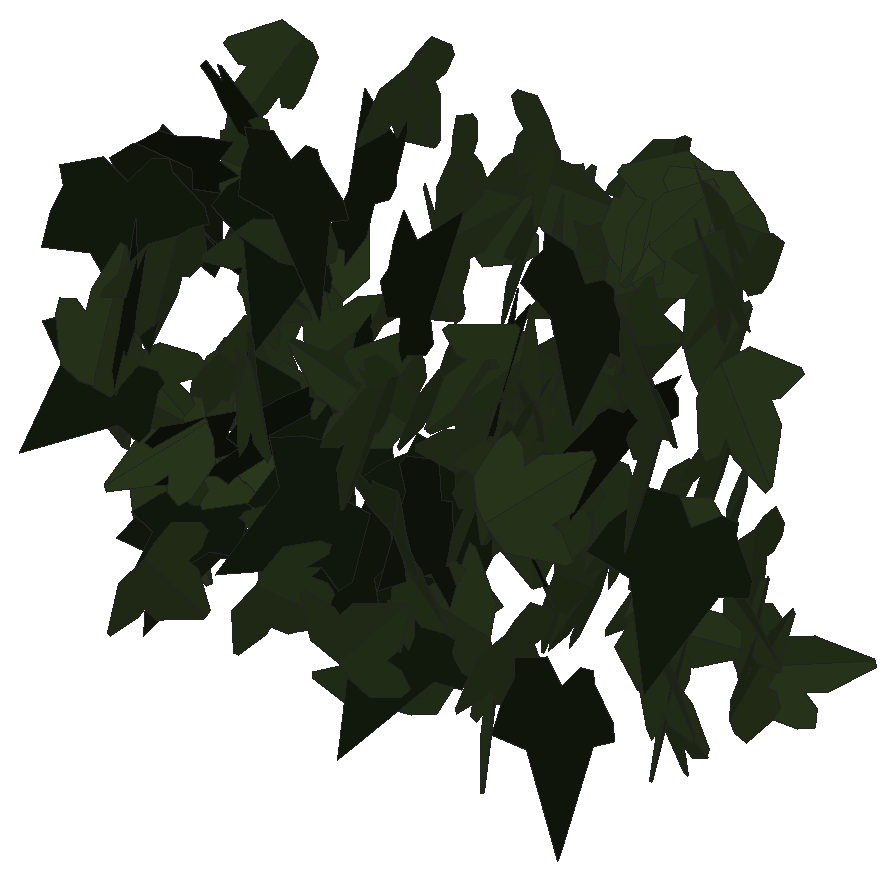
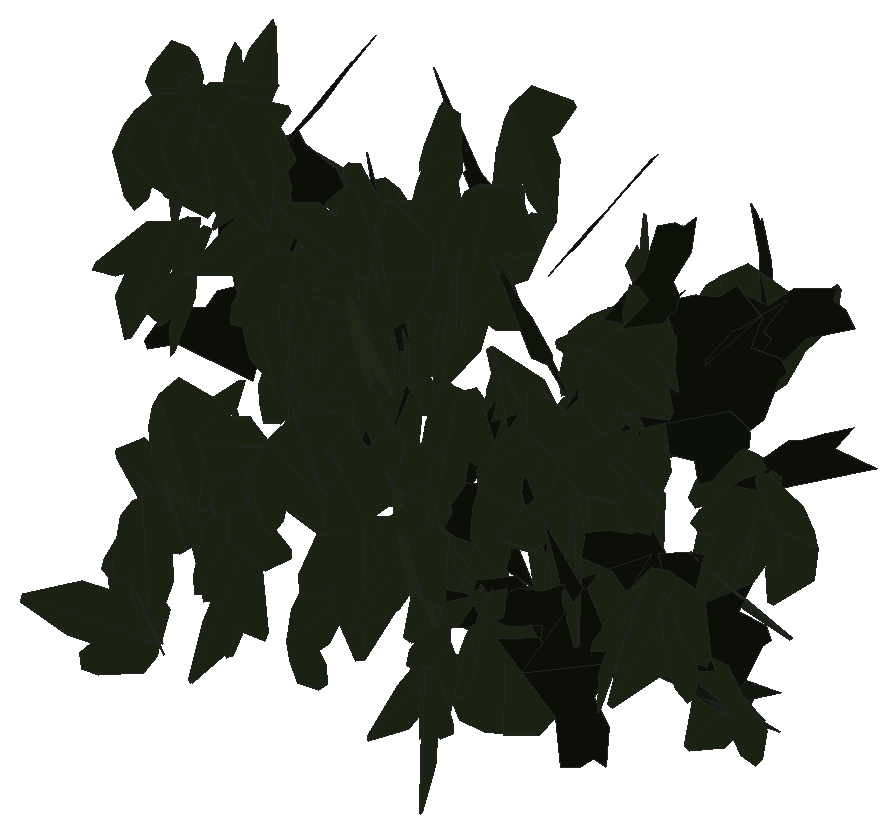
# SketchUp Ruby script. Lengths in inches.
U = 1.inch
M = Sketchup.active_model
def pt(a) = Geom::Point3d.new(a.map { |v| v * U })
def face(e, loops, mat)
  f = e.add_face(loops[0].map { |a| pt(a) })
  loops[1..].each { |l| e.add_face(l.map { |a| pt(a) }).erase! }
  f.material = f.back_material = mat if mat
  f
end
# faces: each face lists its corners as indices into pts; further lists are holes
def faces(e, pts, list, mat = nil) = list.each { |f| face(e, (f[0].is_a?(Array) ? f : [f]).map { |l| l.map { |i| pts[i] } }, mat) }
# xy, xz, yz: faces in a plane at the given z, y or x. An outline is a flat list of corners, or four numbers for a rectangle; further outlines are holes
def ring(l) = l.size == 4 ? [[l[0], l[1]], [l[2], l[1]], [l[2], l[3]], [l[0], l[3]]] : l.each_slice(2).to_a
def flat(e, list, mat, &to3) = list.each { |f| face(e, (f[0].is_a?(Array) ? f : [f]).map { |l| ring(l).map { |u, v| to3.(u, v) } }, mat) }
def xy(e, z, list, mat = nil) = flat(e, list, mat) { |x, y| [x, y, z] }
def xz(e, y, list, mat = nil) = flat(e, list, mat) { |x, z| [x, y, z] }
def yz(e, x, list, mat = nil) = flat(e, list, mat) { |y, z| [x, y, z] }
def lines(e, pts, list) = list.each { |a, b| e.add_line(pt(pts[a]), pt(pts[b])) }
# prism: a flat outline (further loops are holes) pulled along v
def prism(e, loops, v, mat = nil)
  f = face(e, loops, mat); d = Geom::Vector3d.new(v.map { |x| x * U })
  f.pushpull(f.normal.samedirection?(d) ? d.length : -d.length)
end
def box(e, o, s, mat = nil) = prism(e, [[o, [o[0] + s[0], o[1], o[2]], [o[0] + s[0], o[1] + s[1], o[2]], [o[0], o[1] + s[1], o[2]]]], [0, 0, s[2]], mat)
def at(x, y, z, deg = 0) = Geom::Transformation.translation(pt([x, y, z])) * Geom::Transformation.rotation(ORIGIN, Z_AXIS, deg.degrees)
def axes(o, x, y, z) = Geom::Transformation.new([*x, 0, *y, 0, *z, 0, *pt(o).to_a, 1])
def part(name) = M.definitions.add(name)
# library, detail: a bought-in or finely detailed component or shape, given as its bounding box
def library(name, o, s) = part(name).tap { |d| box(d.entities, o, s) }
def detail(e, o, s) = box(e.add_group.entities, o, s)
def put(e, d, t, mat = nil) = e.add_instance(d, t).tap { |i| i.material = mat if mat }
def group(e, t, mat = nil) = e.add_group.tap { |g| g.transformation = t; g.material = mat if mat }.entities
root = M.entities
M.materials.add("efeu1").color = [18, 25, 13]
M.materials.add("efeu2").color = [43, 57, 29]
c1 = part("ivyleaf_10")
p = [[0,0.5,-0.03],[-0.0625,2.02,-0.43],[-0.19,2.01,-0.46],[-0.54,1.05,-0.29],[-0.52,0.625,-0.18],[-0.83,0.76,-0.28],
  [-1.16,0.64,-0.33],[-1.15,0.33,-0.24],[-0.77,-0.39,0.02],[-0.3,-0.51,0.16],[0.04,-0.48,0.23],[-0.02,2.01,-0.4375],
  [-0.06,2.01,-0.43],[0.04,-0.49,0.23],[0.67,-0.49,0.14],[1.38,0.36,-0.2],[1.375,0.51,-0.24],[0.81,0.65,-0.19],
  [0.62,0.59,-0.15],[0.6,1.09,-0.28],[0.5,1.23,-0.31]]
faces(c1.entities,p,[[0,1,2,3,4,5,6,7,8,9,10],[11,12,0,13,14,15,16,17,18,19,20]],"efeu2")
c2 = part("ivyleaf_9")
p = [[1.54,2.16,1.25],[1.36,2.04,1.19],[-0.21,0.99,0.68],[-0.71,1.11,0.82],[-0.85,0.86,0.67],[-0.8,0.17,0.21],
  [-0.9,-0.01,0.1],[-0.67,-0.16,-0.02],[-0.08,-0.08,-0.05],[-0.03,-0.6,-0.4],[0.65,-0.88,-0.66],[0.83,-0.6,-0.49],
  [1.29,-0.42,-0.43],[1.8125,-0.07,-0.26],[1.21,0.44,0.15]]
faces(c2.entities,p,[[0,1,2,3,4,5,6,7,8,9,10,11,12,13,14]],"efeu1")
put(root,c1,axes([9.7,225.84,206.36],[-0.10832,-0.28238,0.32794],[-0.00036,-0.324,-0.30187],[0.45714,-0.06717,0.07747]))
put(root,c1,axes([9.29,223.8125,203.9],[-0.03128,0.02173,-0.49855],[0.46376,-0.18318,-0.03708],[-0.18425,-0.46473,-0.00869]))
put(root,c2,axes([9.76,223.5,204.3],[-0.26977,-0.28177,0.22652],[-0.12075,-0.19055,-0.38971],[0.36518,-0.27115,0.03847]))
put(root,c2,axes([9.46,224.26,205.93],[0.38525,0.18712,0.17078],[0.1531,0.08321,-0.41886],[-0.22103,0.38378,0.00754]))
put(root,c1,axes([9.39,224.5,202.49],[0.33537,-0.04152,0.31386],[0.32897,0.0364,-0.32075],[0.00452,0.43148,0.05726]))
put(root,c1,axes([9.6875,223.63,204.17],[0.14141,-0.25835,-0.33754],[0.03427,0.34558,-0.27278],[0.4467,0.05528,0.12778]))
put(root,c1,axes([9.69,225.07,203.64],[-0.13564,-0.34005,-0.34054],[0.1149,0.3207,-0.36599],[0.46733,-0.17754,-0.00886]))
put(root,c1,axes([9.63,223.86,203.98],[-0.29571,-0.23355,-0.25413],[0.21056,0.14777,-0.37408],[0.29822,-0.33592,0.01213]))
put(root,c1,axes([10.03,224.08,203.4],[-0.31744,0.24813,0.21126],[-0.34629,-0.22324,-0.1989],[-0.00523,-0.27896,0.34709]))
put(root,c2,axes([9.47,224.44,205.375],[0.39903,-0.16624,0.1647],[0.16336,-0.04948,-0.42104],[0.18655,0.39893,0.0164]))
put(root,c2,axes([9.79,224.36,205.67],[-0.12444,-0.40057,0.27214],[-0.06881,-0.26351,-0.41932],[0.47935,-0.14181,0.01046]))
put(root,c1,axes([9.53,225.17,203.38],[0.27389,-0.0933,0.35453],[0.37158,-0.03084,-0.27497],[0.08735,0.42376,0.05804]))
put(root,c2,axes([9.7,223.63,205.99],[-0.14197,-0.4208,-0.22972],[0.09472,0.21024,-0.44365],[0.46997,-0.16949,0.02002]))
put(root,c1,axes([9.84,225.4,203.71],[-0.16225,0.45566,0.12667],[-0.04203,0.11949,-0.48369],[-0.47107,-0.1676,-0.00048]))
put(root,c2,axes([9.71,224.12,203.13],[0.30447,0.20798,0.26818],[0.20224,0.17927,-0.36329],[-0.29515,0.33739,0.02771]))
put(root,c2,axes([10.03,224.42,202.54],[-0.43075,-0.13322,-0.11581],[0.18043,-0.21842,-0.35054],[0.0511,-0.35181,0.26149]))
put(root,c2,axes([9.91,224.43,202.41],[-0.35805,-0.24256,-0.14882],[0.26708,-0.14498,-0.34027],[0.14553,-0.33071,0.25832]))
put(root,c1,axes([10.21,222.53,204.96],[0.07198,0.37465,-0.3232],[0.01875,0.3243,0.3801],[0.49444,-0.06684,0.03263]))
put(root,c2,axes([9.97,224.7,206.62],[0.39797,-0.30186,0.02239],[0.01577,-0.01625,-0.49949],[0.30227,0.39827,-0.00342]))
put(root,c1,axes([10.37,223.37,205.67],[-0.07272,-0.49292,0.04169],[-0.00779,-0.04099,-0.49826],[0.49462,-0.07311,-0.00171]))
put(root,c1,axes([10.04,224.91,204.64],[-0.11638,-0.06495,0.48191],[0.48351,-0.06818,0.10758],[0.05174,0.49105,0.07868]))
put(root,c1,axes([10.125,224.65,202.82],[-0.17416,-0.26781,-0.31458],[0.43295,-0.14648,-0.0874],[-0.05412,-0.30992,0.31315]))
put(root,c1,axes([10.08,224.77,205.79],[0.02851,-0.01874,0.49883],[0.47672,0.14924,-0.02164],[-0.14808,0.47684,0.02638]))
put(root,c2,axes([10.66,222.375,205.32],[-0.02342,0.11384,0.4863],[-0.05898,0.4828,-0.11586],[-0.49596,-0.06279,-0.00918]))
put(root,c2,axes([10.34,224.49,203.25],[0.22993,0.28852,0.33748],[0.21471,0.2604,-0.36891],[-0.38863,0.31457,-0.00414]))
put(root,c1,axes([10.76,225.13,204.83],[0.31324,0.11014,0.37383],[-0.3639,-0.08901,0.33114],[0.13949,-0.47953,0.0244]))
put(root,c1,axes([10.2,225.04,203.39],[0.35907,0.04494,0.34503],[0.34411,0.02753,-0.3617],[-0.05151,0.49721,-0.01115]))
put(root,c1,axes([10.86,225,203.92],[-0.29967,0.17096,0.3619],[-0.32155,0.16638,-0.34485],[-0.23834,-0.43942,0.01022]))
put(root,c1,axes([10.88,224.34,205.59],[-0.26864,-0.41556,0.07168],[-0.02912,-0.06651,-0.4947],[0.42069,-0.26997,0.01154]))
put(root,c2,axes([10.66,224.65,205.59],[-0.0311,-0.45326,0.20879],[0.00758,-0.2096,-0.45389],[0.49897,-0.02507,0.01991]))
put(root,c2,axes([11.1,224.99,202.9375],[-0.37001,-0.33248,-0.0505],[-0.03738,-0.03395,0.49744],[-0.33421,0.37189,0.00026]))
put(root,c2,axes([11.12,224.99,203.64],[-0.06882,0.13569,0.47629],[-0.20573,0.42958,-0.15211],[-0.45049,-0.21691,-0.0033]))
put(root,c1,axes([10.875,224.91,204.22],[0.04692,0.01713,-0.4975],[0.11586,0.4856,0.02765],[0.48412,-0.11788,0.04159]))
put(root,c2,axes([10.63,224.98,202.35],[0.221,-0.07486,-0.44221],[0.44046,0.12921,0.19825],[0.0846,-0.47718,0.12306]))
put(root,c1,axes([11.04,222.33,203.22],[-0.12281,-0.37526,-0.30675],[0.11594,0.28451,-0.39448],[0.47061,-0.16801,0.01713]))
put(root,c2,axes([11.44,224.91,205.93],[-0.34057,0.15532,-0.3315],[-0.31036,0.1176,0.37396],[0.19413,0.46049,0.01631]))
put(root,c1,axes([11.61,224.84,203.9],[-0.26757,-0.01755,-0.42202],[-0.41877,-0.05418,0.26776],[-0.05513,0.49675,0.01429]))
put(root,c1,axes([11.49,226.18,202.57],[0.15407,-0.39205,-0.26937],[-0.04768,0.26899,-0.41877],[0.47327,0.15473,0.0455]))
put(root,c1,axes([11.6,223.98,203.13],[-0.22631,-0.3645,0.25676],[-0.13604,-0.21776,-0.42904],[0.42459,-0.26405,-0.00061]))
put(root,c2,axes([11.24,224.01,206.59],[0.13693,-0.47655,0.06441],[0.02721,-0.05919,-0.49574],[0.48012,0.13927,0.00973]))
put(root,c1,axes([11.51,225.16,204.09],[-0.03115,-0.29201,0.40467],[0.06812,-0.40415,-0.28639],[0.49436,0.03729,0.06496]))
put(root,c1,axes([11.55,225.28,207.01],[-0.07208,-0.44698,-0.21216],[0.05964,0.20499,-0.45213],[0.49117,-0.09049,0.02377]))
put(root,c2,axes([11.95,223.84,203.52],[-0.2257,-0.27373,0.35232],[-0.20472,-0.28728,-0.35435],[0.39642,-0.30421,0.0176]))
put(root,c1,axes([11.91,225.53,202.48],[0.01948,-0.18418,-0.46443],[0.10604,0.45572,-0.17628],[0.48824,-0.09163,0.05681]))
put(root,c1,axes([11.88,222.93,203.03],[-0.17271,-0.2765,-0.3791],[0.18195,0.33289,-0.3257],[0.43251,-0.25046,-0.01437]))
put(root,c1,axes([11.65,222.88,205.09],[0.08422,-0.04811,0.4905],[0.43437,-0.22788,-0.09693],[0.23288,0.44244,0.00341]))
put(root,c1,axes([12.13,224.32,201.46],[-0.42741,-0.25897,-0.01587],[-0.00996,-0.01418,0.4997],[-0.25927,0.42747,0.00697]))
put(root,c2,axes([12.47,223.58,203.07],[-0.32905,0.302,0.22478],[-0.16852,0.1488,-0.44661],[-0.33664,-0.36967,0.00387]))
put(root,c1,axes([12.29,224.79,204.5],[-0.01566,-0.39834,-0.30179],[-0.00759,0.3021,-0.39835],[0.4997,-0.0079,-0.01551]))
put(root,c1,axes([12.22,225.43,203.57],[-0.06506,-0.27499,-0.41249],[0.11942,0.39508,-0.28222],[0.48115,-0.13524,0.01428]))
put(root,c1,axes([12.31,224.54,205.74],[-0.11911,-0.41076,-0.25901],[0.05981,0.25225,-0.42754],[0.48191,-0.13283,-0.01095]))
put(root,c1,axes([12.34,225.33,203.59],[0.17201,-0.46737,0.04451],[0.01584,-0.04159,-0.49802],[0.46922,0.17273,0.0005]))
put(root,c1,axes([12.42,224.78,205.47],[-0.33759,0.3666,-0.04042],[-0.03196,0.02551,0.49833],[0.36744,0.33904,0.00621]))
put(root,c1,axes([12.34,224.57,201.87],[-0.1633,0.36197,0.30383],[0.12667,-0.27617,0.39709],[0.45529,0.20666,-0.00151]))
put(root,c2,axes([12.46,224.28,202.39],[-0.40294,-0.29381,-0.03626],[0.02905,0.02171,-0.49868],[0.29461,-0.40399,-0.00043]))
put(root,c2,axes([12.5625,224.58,203.48],[-0.45434,-0.20009,-0.05947],[0.05551,0.02149,-0.49644],[0.20122,-0.45772,0.00268]))
put(root,c1,axes([12.56,225.18,205.98],[0.02545,-0.1364,0.48036],[0.01344,0.481,0.13587],[-0.49917,0.006,0.02815]))
put(root,c1,axes([12.63,225.69,205.82],[0.21022,-0.41929,0.17322],[0.07286,-0.15723,-0.46901],[0.44777,0.22243,-0.005]))
put(root,c1,axes([12.62,224.26,202.75],[-0.45914,0.00374,-0.19792],[0.19796,0.00596,-0.45911],[-0.00107,-0.49995,-0.00695]))
put(root,c1,axes([12.91,225.41,206.79],[0.27547,-0.25082,-0.33348],[-0.22269,0.24957,-0.37165],[0.35289,0.35328,0.02579]))
put(root,c1,axes([12.79,224.375,206.99],[0.12208,-0.37229,-0.31064],[0.06112,0.32959,-0.37099],[0.481,0.0526,0.12598]))
put(root,c2,axes([12.64,224.32,203.54],[0.14201,-0.1982,-0.43652],[0.31313,-0.3064,0.24098],[-0.36302,-0.34182,0.0371]))
put(root,c1,axes([12.89,225.36,203.22],[-0.35078,-0.35628,0.00439],[-0.00072,-0.00545,-0.49997],[0.3563,-0.35077,0.00331]))
put(root,c1,axes([12.81,224.3,206.34],[0.03806,-0.08742,-0.49083],[0.07965,0.487,-0.08056],[0.49215,-0.07206,0.05099]))
put(root,c1,axes([12.76,224.85,203.55],[0.14992,-0.34298,0.33149],[0.12562,-0.30682,-0.37427],[0.46015,0.19551,-0.00583]))
put(root,c1,axes([13.23,224.14,202.59],[0.00159,0.04982,0.49751],[-0.49929,0.02667,-0.00108],[-0.02664,-0.4968,0.04983]))
put(root,c2,axes([12.77,223.67,205.8125],[-0.13981,0.28282,0.3879],[0.16759,-0.34985,0.31547],[0.44985,0.21822,0.00303]))
put(root,c1,axes([13.07,225.625,205.8],[-0.13826,0.26404,0.40145],[-0.18964,0.35385,-0.29804],[-0.4415,-0.23468,0.0023]))
put(root,c1,axes([13.05,225.33,203.66],[-0.16028,-0.45346,0.1367],[0.05069,0.12706,0.48092],[-0.47089,0.16802,0.00524]))
put(root,c1,axes([12.79,225.64,206.23],[-0.10789,-0.01062,0.4881],[0.48783,0.01765,0.10822],[-0.01953,0.49958,0.00656]))
put(root,c1,axes([13.26,225.97,204.25],[-0.0713,-0.39766,0.29459],[0.03186,-0.3007,-0.3982],[0.49386,-0.03801,0.06822]))
put(root,c1,axes([13.04,222.58,202.93],[-0.38161,-0.09527,0.3087],[0.30148,0.0667,0.39327],[-0.11611,0.48629,0.00654]))
put(root,c1,axes([12.94,223.42,203.35],[-0.02447,-0.00915,0.49932],[0.47654,-0.14994,0.02061],[0.14936,0.4769,0.01606]))
put(root,c1,axes([13.15,225.89,204.64],[0.29494,-0.26113,0.30792],[0.24603,-0.18611,-0.39349],[0.32012,0.38363,0.01871]))
put(root,c1,axes([13.71,225.125,203.89],[-0.14383,-0.06173,0.47487],[-0.43401,-0.19271,-0.15651],[0.20235,-0.45722,0.00185]))
put(root,c1,axes([13.23,225.76,202.4],[0.03549,-0.06347,0.49468],[0.24157,-0.43169,-0.07272],[0.43633,0.24416,0.00002]))
put(root,c1,axes([13.46,224.53,204.33],[-0.0981,-0.4544,0.1841],[-0.02189,-0.18351,-0.46459],[0.48979,-0.09921,0.01611]))
put(root,c1,axes([13.4,224.11,204.51],[-0.29395,-0.39953,-0.06304],[-0.02421,-0.0604,0.49575],[-0.40374,0.2945,0.01616]))
put(root,c1,axes([13.68,224.11,205.4375],[-0.18228,-0.26081,0.38569],[-0.20753,-0.32526,-0.31802],[0.41678,-0.27602,0.01033]))
put(root,c2,axes([13.32,224.3,204.94],[-0.03418,0.2861,0.40863],[0.04165,-0.40652,0.28811],[0.49709,0.05373,0.00395]))
put(root,c1,axes([13.59,222.22,205.79],[0.07662,-0.47893,0.12148],[0.03153,-0.11794,-0.48487],[0.49309,0.08196,0.01213]))
put(root,c1,axes([13.64,225.39,205.66],[-0.29948,-0.39682,-0.05333],[0.02817,0.04555,-0.49712],[0.39939,-0.30077,-0.00492]))
put(root,c1,axes([13.67,226.16,202.98],[-0.01602,-0.32883,-0.37632],[0.04332,0.37418,-0.32881],[0.49786,-0.04314,0.0165]))
put(root,c1,axes([13.76,224.6,203.12],[0.09068,-0.27678,-0.40641],[-0.02069,0.41075,-0.28435],[0.49127,0.06839,0.06304]))
put(root,c1,axes([14.04,223.92,205.31],[0.00276,0.0001,0.49999],[-0.4715,0.16636,0.00257],[-0.16636,-0.47151,0.00101]))
put(root,c1,axes([13.67,222.35,204.53],[-0.40078,0.07044,0.29054],[0.2631,-0.14766,0.39872],[0.14197,0.47248,0.0813]))
put(root,c1,axes([13.8,224.6,204.79],[-0.19754,-0.39503,-0.23438],[0.11981,0.20199,-0.44141],[0.44343,-0.23055,0.01485]))
put(root,c1,axes([13.9,224.51,205.49],[-0.14506,-0.45615,-0.14453],[0.03156,0.14158,-0.4785],[0.47745,-0.14794,-0.01228]))
put(root,c1,axes([14.15,225.26,205.07],[-0.21164,0.19567,-0.40856],[-0.29269,0.28512,0.28817],[0.34575,0.36114,-0.00614]))
put(root,c2,axes([13.61,224.22,203.7],[0.1068,-0.21926,0.43648],[0.18297,-0.39631,-0.24385],[0.4529,0.21181,-0.00442]))
put(root,c1,axes([13.8,223.64,202.52],[0.31595,-0.29514,0.25113],[0.20386,-0.14897,-0.43157],[0.32957,0.3751,0.0262]))
put(root,c1,axes([14.1,223.41,204.76],[0.11037,-0.29798,0.38604],[-0.1395,0.35997,0.31774],[-0.46729,-0.17784,-0.00367]))
put(root,c1,axes([14.16,225.59,206.96],[0.02798,-0.46498,0.18168],[0.04893,-0.17853,-0.46447],[0.49681,0.04377,0.03551]))
put(root,c1,axes([14.26,225.49,202.86],[-0.05015,-0.48867,-0.09323],[0.01304,0.09238,-0.49122],[0.49731,-0.0517,0.00348]))
put(root,c1,axes([14.18,224.14,203.96],[0.40406,-0.2937,0.02171],[-0.01757,0.01275,0.49953],[-0.29398,-0.40445,-0.00001]))
put(root,c1,axes([14.1875,224.99,205.95],[0.01373,-0.11293,-0.48689],[0.17809,0.45621,-0.10079],[0.46701,-0.17065,0.05275]))
put(root,c1,axes([14.51,222.97,203.36],[-0.07753,-0.43924,-0.22597],[0.04987,0.2206,-0.44592],[0.49143,-0.09169,0.0096]))
put(root,c1,axes([14.54,226,204.1875],[0.10124,-0.48658,0.05471],[0.01515,-0.05273,-0.49698],[0.48941,0.10228,0.00406]))
put(root,c1,axes([14.64,225.41,206.91],[-0.21623,-0.27655,0.35604],[-0.04792,-0.37854,-0.32312],[0.44827,-0.17386,0.1372]))
put(root,c1,axes([14.53,224.55,204.03],[-0.06635,-0.03164,0.49457],[0.26457,-0.42418,0.00835],[0.41905,0.26281,0.07303]))
put(root,c2,axes([14.5,224.04,206.49],[0.04231,-0.45357,0.20611],[0.02389,-0.20476,-0.45552],[0.49763,0.04839,0.00434]))
put(root,c1,axes([14.41,224.97,206.43],[0.36783,0.04175,-0.3361],[0.33483,0.02973,0.37014],[0.05089,-0.49737,-0.00608]))
put(root,c1,axes([14.75,226.07,203.09],[-0.01371,-0.49233,-0.08619],[0.01056,0.08591,-0.49245],[0.4997,-0.01532,0.00804]))
put(root,c1,axes([14.99,225.48,206.75],[-0.25787,-0.1116,0.41358],[-0.1902,-0.40272,-0.22725],[0.38384,-0.27453,0.16525]))
put(root,c1,axes([14.85,225.28,203.5],[-0.07938,-0.15975,0.4671],[0.05071,-0.47323,-0.15323],[0.49105,0.02304,0.09133]))
put(root,c1,axes([14.9,225.25,205.23],[0.05213,0.08229,-0.49042],[-0.02291,0.49298,0.08028],[0.49675,0.0141,0.05517]))
put(root,c1,axes([14.89,225.68,203.69],[0.24411,-0.43593,0.01941],[0.01166,-0.01572,-0.49962],[0.43621,0.24437,0.00249]))
put(root,c1,axes([14.55,222.93,204.79],[0.31802,-0.01261,-0.38562],[0.38576,0.0199,0.31748],[0.00734,-0.49944,0.02239]))
put(root,c1,axes([14.99,224.14,206.07],[0.06073,-0.22247,-0.44364],[0.02174,0.44771,-0.22154],[0.49582,0.00762,0.06405]))
put(root,c1,axes([14.83,226.07,202.51],[0.30413,-0.29439,0.26616],[0.1807,-0.19583,-0.42308],[0.35335,0.35353,-0.01273]))
put(root,c2,axes([15.14,223.79,205.54],[-0.09593,0.43665,-0.22391],[0.04944,-0.21839,-0.44706],[-0.48821,-0.10792,-0.00128]))
put(root,c1,axes([14.83,224.65,202.97],[-0.14805,-0.18122,-0.44186],[0.33208,0.2934,-0.2316],[0.34323,-0.36204,0.03348]))
put(root,c1,axes([14.73,224.95,202.06],[-0.01956,0.04217,-0.49783],[0.3577,-0.34665,-0.04341],[-0.34881,-0.35784,-0.01661]))
put(root,c1,axes([15.06,225.16,207.07],[-0.41479,0.27816,-0.024],[0.01919,-0.01446,-0.49942],[-0.27853,-0.41523,0.00132]))
put(root,c1,axes([14.98,224.73,202.55],[0.30291,-0.32331,0.23176],[0.15077,-0.17627,-0.44294],[0.36813,0.33823,-0.0093]))
put(root,c1,axes([15.27,224.9,206.64],[-0.41611,0.22146,0.16675],[-0.14993,0.0732,-0.47134],[-0.23317,-0.44227,0.00549]))
put(root,c1,axes([15.27,225.34,206.55],[-0.10127,-0.41239,0.26397],[-0.05535,-0.25819,-0.42459],[0.4865,-0.11522,0.00664]))
put(root,c1,axes([15.07,224.31,205.04],[0.13321,-0.28827,0.38621],[0.22896,-0.31472,-0.31389],[0.42407,0.26048,0.04816]))
put(root,c1,axes([14.95,226.01,201.94],[-0.10524,-0.06697,0.48419],[0.38302,0.29641,0.12425],[-0.30368,0.39706,-0.01109]))
put(root,c1,axes([14.93,224.48,202.68],[0.0799,-0.0451,0.49151],[0.46715,-0.15383,-0.09006],[0.15934,0.47361,0.01756]))
put(root,c1,axes([15.42,225.2,202.16],[0.0978,-0.20584,0.44504],[-0.20126,0.39697,0.22784],[-0.44713,-0.2237,-0.00521]))
put(root,c2,axes([15.32,222.69,203.29],[-0.33881,-0.12372,-0.34627],[0.32657,0.11514,-0.36068],[0.16899,-0.47057,0.00279]))
put(root,c1,axes([15.36,225.07,205.31],[0.07885,0.47487,0.1352],[0.02247,0.13332,-0.48138],[-0.49323,0.08199,-0.00032]))
put(root,c1,axes([15.14,225.33,202.95],[-0.00869,-0.07269,0.49461],[0.48269,-0.12998,-0.01062],[0.13013,0.47731,0.07243]))
put(root,c2,axes([15.47,224.3,204.24],[-0.25294,-0.42803,-0.05304],[0.02439,0.04719,-0.49717],[0.43061,-0.2541,-0.00299]))
put(root,c1,axes([15.68,223.58,205.81],[-0.43513,0.21157,-0.12608],[-0.11344,0.05504,0.48384],[0.21861,0.44968,0.0001]))
